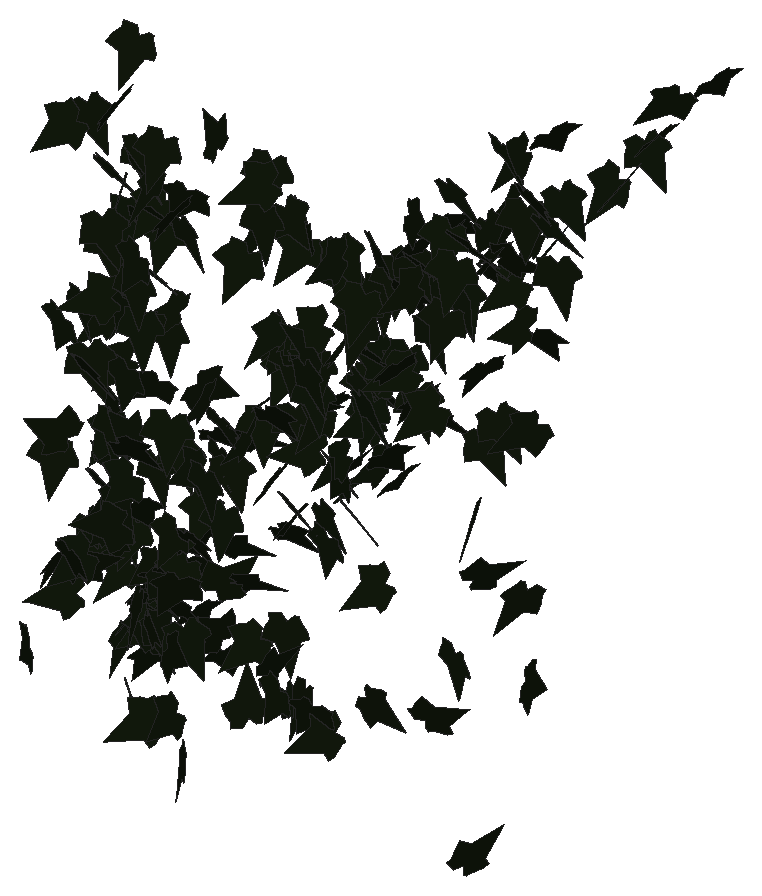
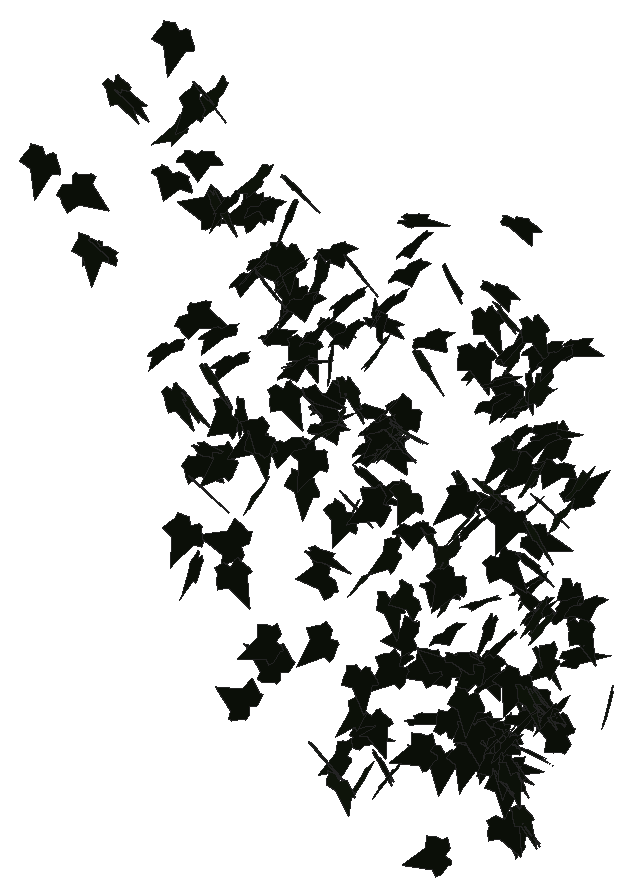
# SketchUp Ruby script. Lengths in inches.
U = 1.inch
M = Sketchup.active_model
def pt(a) = Geom::Point3d.new(a.map { |v| v * U })
def face(e, loops, mat)
  f = e.add_face(loops[0].map { |a| pt(a) })
  loops[1..].each { |l| e.add_face(l.map { |a| pt(a) }).erase! }
  f.material = f.back_material = mat if mat
  f
end
# faces: each face lists its corners as indices into pts; further lists are holes
def faces(e, pts, list, mat = nil) = list.each { |f| face(e, (f[0].is_a?(Array) ? f : [f]).map { |l| l.map { |i| pts[i] } }, mat) }
# xy, xz, yz: faces in a plane at the given z, y or x. An outline is a flat list of corners, or four numbers for a rectangle; further outlines are holes
def ring(l) = l.size == 4 ? [[l[0], l[1]], [l[2], l[1]], [l[2], l[3]], [l[0], l[3]]] : l.each_slice(2).to_a
def flat(e, list, mat, &to3) = list.each { |f| face(e, (f[0].is_a?(Array) ? f : [f]).map { |l| ring(l).map { |u, v| to3.(u, v) } }, mat) }
def xy(e, z, list, mat = nil) = flat(e, list, mat) { |x, y| [x, y, z] }
def xz(e, y, list, mat = nil) = flat(e, list, mat) { |x, z| [x, y, z] }
def yz(e, x, list, mat = nil) = flat(e, list, mat) { |y, z| [x, y, z] }
def lines(e, pts, list) = list.each { |a, b| e.add_line(pt(pts[a]), pt(pts[b])) }
# prism: a flat outline (further loops are holes) pulled along v
def prism(e, loops, v, mat = nil)
  f = face(e, loops, mat); d = Geom::Vector3d.new(v.map { |x| x * U })
  f.pushpull(f.normal.samedirection?(d) ? d.length : -d.length)
end
def box(e, o, s, mat = nil) = prism(e, [[o, [o[0] + s[0], o[1], o[2]], [o[0] + s[0], o[1] + s[1], o[2]], [o[0], o[1] + s[1], o[2]]]], [0, 0, s[2]], mat)
def at(x, y, z, deg = 0) = Geom::Transformation.translation(pt([x, y, z])) * Geom::Transformation.rotation(ORIGIN, Z_AXIS, deg.degrees)
def axes(o, x, y, z) = Geom::Transformation.new([*x, 0, *y, 0, *z, 0, *pt(o).to_a, 1])
def part(name) = M.definitions.add(name)
# library, detail: a bought-in or finely detailed component or shape, given as its bounding box
def library(name, o, s) = part(name).tap { |d| box(d.entities, o, s) }
def detail(e, o, s) = box(e.add_group.entities, o, s)
def put(e, d, t, mat = nil) = e.add_instance(d, t).tap { |i| i.material = mat if mat }
def group(e, t, mat = nil) = e.add_group.tap { |g| g.transformation = t; g.material = mat if mat }.entities
root = M.entities
M.materials.add("efeu1").color = [18, 25, 13]
c1 = part("ivyleaf_9")
p = [[1.54,2.16,1.25],[1.36,2.04,1.19],[-0.21,0.99,0.68],[-0.71,1.11,0.82],[-0.85,0.86,0.67],[-0.8,0.17,0.21],
  [-0.9,-0.01,0.1],[-0.67,-0.16,-0.02],[-0.08,-0.08,-0.05],[-0.03,-0.6,-0.4],[0.65,-0.88,-0.66],[0.83,-0.6,-0.49],
  [1.29,-0.42,-0.43],[1.8125,-0.07,-0.26],[1.21,0.44,0.15]]
faces(c1.entities,p,[[0,1,2,3,4,5,6,7,8,9,10,11,12,13,14]],"efeu1")
put(root,c1,axes([656.24,122.11,335.02],[-0.71022,1.11665,-0.15151],[0.0503,-0.14751,-1.32287],[-1.12576,-0.71106,0.03648]))
put(root,c1,axes([656.28,114.59,383.84],[-1.00018,-0.83735,0.69377],[-0.54915,-0.42464,-1.3042],[0.93857,-1.14077,-0.02376]))
put(root,c1,axes([655.3125,117.78,345.35],[0.65695,-1.07778,-0.75279],[-0.21372,0.74279,-1.24998],[1.29716,0.66822,0.1753]))
put(root,c1,axes([655.89,121.85,333.43],[-1.01827,-0.15161,-0.85733],[0.8683,-0.27334,-0.98296],[-0.06368,-1.30275,0.30601]))
put(root,c1,axes([655.37,116.96,366.04],[0.34286,-1.26926,0.60559],[0.26805,-0.55292,-1.31063],[1.38055,0.42258,0.10408]))
put(root,c1,axes([655.04,116.78,341.77],[0.99807,0.54618,-0.89303],[0.59041,0.7252,1.10339],[0.86443,-1.12594,0.27748]))
put(root,c1,axes([655.93,112.92,354.41],[-0.44767,-1.43357,-0.10005],[0.02948,0.09561,-1.50184],[1.43676,-0.44864,-0.00035]))
put(root,c1,axes([656.02,116.79,384.34],[0.25998,-1.28733,-0.70574],[-0.04875,0.70875,-1.31079],[1.46728,0.25164,0.08149]))
put(root,c1,axes([656.93,118.92,345],[-1.19552,-0.67601,0.07235],[-0.03238,-0.08956,-1.37202],[0.6791,-1.19436,0.06194]))
put(root,c1,axes([655.97,119.44,356.38],[1.06878,-0.9039,-0.24977],[-0.2235,0.12227,-1.39886],[0.91075,1.09074,-0.05018]))
put(root,c1,axes([657.5,117.57,345.86],[-1.23788,0.59991,-0.12376],[0.09621,-0.08516,-1.37516],[-0.60494,-1.24114,0.03453]))
put(root,c1,axes([656.03,134.68,335.79],[1.07083,0.22816,0.82919],[0.79435,0.24505,-1.09327],[-0.32956,1.33199,0.0591]))
put(root,c1,axes([658.09,117.64,345.03],[-0.32565,0.33631,-1.32818],[-1.11303,-0.86102,0.05488],[-0.79895,1.06242,0.46491]))
put(root,c1,axes([656.29,117.14,350.09],[1.35102,-0.32608,-0.00191],[-0.00104,0.00383,-1.38981],[0.32608,1.35102,0.00348]))
put(root,c1,axes([657.69,118.04,345.98],[-1.08082,0.8425,-0.16461],[0.12152,-0.11184,-1.37033],[-0.84978,-1.08755,0.0134]))
put(root,c1,axes([657.45,120.125,340.79],[-1.34084,-0.32062,-0.13981],[0.2222,-0.35305,-1.32142],[0.27012,-1.30105,0.39303]))
put(root,c1,axes([657.78,119.51,346.84],[-0.73022,1.16159,0.10689],[-0.05352,0.09262,-1.37204],[-1.16527,-0.73217,-0.00397]))
put(root,c1,axes([657.84,118.625,364.92],[-1.13991,0.87237,0.01427],[0.01406,0.04184,-1.43481],[-0.87238,-1.13923,-0.04177]))
put(root,c1,axes([656.69,120.92,344.59],[0.29639,-1.33638,-0.06778],[0.00877,0.07137,-1.36864],[1.33807,0.29555,0.02398]))
put(root,c1,axes([657.06,112.25,366.8],[-0.12136,-1.0892,1.01192],[0.30145,-1.01222,-1.05337],[1.45584,0.1188,0.30247]))
put(root,c1,axes([658.18,121.28,338.84],[-0.39023,1.27902,-0.09719],[0.01077,-0.09831,-1.33709],[-1.28266,-0.38995,0.01834]))
put(root,c1,axes([657.43,107.34,338.91],[0.04723,-0.43721,1.3925],[0.06038,-1.39145,-0.43893],[1.45827,0.07177,-0.02692]))
put(root,c1,axes([657.91,120.46,344.6],[-0.77173,-1.13212,-0.03722],[0.04554,0.01399,-1.36981],[1.13182,-0.7725,0.02973]))
put(root,c1,axes([658.65,115.96,349.41],[-0.98779,0.96189,-0.18111],[0.13218,-0.12386,-1.37875],[-0.96982,-0.99659,-0.00345]))
put(root,c1,axes([657.99,117.75,354.74],[-0.54169,-1.13622,0.61477],[-0.15612,-0.60416,-1.25418],[1.28241,-0.55349,0.107]))
put(root,c1,axes([658.32,121.66,337.93],[0.48242,1.21405,-0.3295],[-0.1248,-0.30497,-1.30638],[-1.25177,0.49829,0.00326]))
put(root,c1,axes([658.9,118.3,361.04],[-1.42192,0.17774,0.05329],[-0.0556,-0.01523,-1.43281],[-0.17703,-1.42283,0.022]))
put(root,c1,axes([657.73,117.9375,355.5],[0.08364,-1.39785,0.08215],[-0.01645,-0.08327,-1.40018],[1.40016,0.08253,-0.02136]))
put(root,c1,axes([659.01,115.96,366.48],[-1.42993,0.25709,-0.07317],[0.04156,-0.17951,-1.44299],[-0.26404,-1.42051,0.16911]))
put(root,c1,axes([658.87,121.53,332.9],[0.01974,1.02003,-0.88375],[-0.14459,-0.87716,-1.01566],[-1.34186,0.10952,0.09644]))
put(root,c1,axes([657.73,116.39,379.9],[1.33733,-0.63028,-0.0417],[0.06152,0.22713,-1.46016],[0.62865,1.31856,0.23159]))
put(root,c1,axes([657.78,116.74,352.91],[0.62527,-1.2148,0.28921],[0.21503,-0.21386,-1.36322],[1.2301,0.65488,0.0913]))
put(root,c1,axes([658.76,122.36,337.74],[-1.09637,-0.26636,-0.72385],[0.74209,-0.02137,-1.11614],[0.21024,-1.31359,0.16494]))
put(root,c1,axes([659.14,121.8,339.61],[0.71264,0.8805,-0.72368],[-0.45012,-0.56669,-1.13274],[-1.04709,0.84287,-0.00559]))
put(root,c1,axes([659.58,116.03,386.12],[-0.62586,1.32112,-0.36173],[0.13171,-0.33782,-1.46166],[-1.3634,-0.63908,0.02485]))
put(root,c1,axes([658.25,134.16,346.49],[1.00881,0.33998,0.83846],[0.7427,0.40602,-1.05823],[-0.51672,1.24734,0.11593]))
put(root,c1,axes([658.53,116.38,373.48],[-0.10525,-1.44792,-0.35467],[0.21802,0.33678,-1.43958],[1.4747,-0.15313,0.18752]))
put(root,c1,axes([659.14,118.82,347.63],[0.94591,0.99244,-0.16489],[-0.11204,-0.121,-1.37101],[-0.99978,0.95252,-0.00236]))
put(root,c1,axes([659.06,121.66,341.04],[0.37215,-0.59504,-1.15024],[0.59763,-0.98283,0.70179],[-1.1489,-0.70399,-0.00753]))
put(root,c1,axes([660.35,119.15,337.49],[-0.9,0.89881,0.43769],[-0.35351,0.26475,-1.27058],[-0.93513,-0.96513,0.05907]))
put(root,c1,axes([658.89,119.1,328.8],[-0.15229,-0.16631,1.41236],[0.40306,-1.36724,-0.11753],[1.3638,0.38551,0.19245]))
put(root,c1,axes([659.97,120.03,341.08],[0.58504,1.21298,-0.06639],[-0.14393,-0.00395,-1.34062],[-1.20624,0.58878,0.12777]))
put(root,c1,axes([660.34,107.78,348.32],[-0.56945,1.20528,-0.58163],[0.25936,-0.52072,-1.33299],[-1.31291,-0.62563,-0.01105]))
put(root,c1,axes([661.02,116.12,355.15],[-0.27991,0.4357,1.38305],[-0.9607,0.99937,-0.50926],[-1.08615,-0.99622,0.09402]))
put(root,c1,axes([661.125,108.58,344.625],[-0.89995,-0.31747,1.08852],[-0.93011,-0.58814,-0.94051],[0.64851,-1.28409,0.16165]))
put(root,c1,axes([661.1,119.17,337.36],[-1.31357,-0.20553,0.30416],[-0.29593,-0.0758,-1.32925],[0.21721,-1.34619,0.02841]))
put(root,c1,axes([660.32,118.36,365.46],[1.02839,0.989,-0.20213],[-0.16985,-0.1149,-1.42636],[-0.99505,1.04175,0.03457]))
put(root,c1,axes([659.83,116.28,368.03],[0.05204,-1.12236,0.94769],[0.22028,-0.9316,-1.1154],[1.45233,0.18151,0.13522]))
put(root,c1,axes([660.18,116.09,378.82],[-0.63713,0.12987,-1.35187],[1.18093,-0.68446,-0.62232],[-0.6707,-1.32854,0.18847]))
put(root,c1,axes([660.57,121.2,340.62],[1.18084,0.30799,-0.57443],[-0.55151,-0.16135,-1.22025],[-0.34736,1.30319,-0.01532]))
put(root,c1,axes([661.71,118.53,360.02],[0.04728,0.67777,-1.2711],[-0.8779,-0.99476,-0.56307],[-1.14209,0.79271,0.38021]))
put(root,c1,axes([660.45,120.5,340.84],[0.5226,-1.11443,-0.62384],[-0.30285,0.54669,-1.23031],[1.24073,0.60284,-0.03755]))
put(root,c1,axes([660.5,119.97,351.72],[0.23802,-1.37389,-0.11875],[-0.00334,0.11993,-1.39425],[1.37901,0.23743,0.01712]))
put(root,c1,axes([661.4375,115.52,376.19],[-0.75501,-0.51266,1.16043],[-0.61135,-1.03622,-0.85555],[1.11161,-0.91809,0.31765]))
put(root,c1,axes([662.24,111.69,370.9],[-0.98534,-0.3661,1.03841],[-0.92225,-0.48682,-1.04675],[0.60148,-1.34618,0.09614]))
put(root,c1,axes([662.32,121.78,342.32],[0.59601,0.91809,-0.79993],[-0.47504,-0.64474,-1.09392],[-1.12121,0.7612,0.03825]))
put(root,c1,axes([662.61,105.65,360.88],[0.06608,0.00927,1.487],[-1.30235,-0.71808,0.06235],[0.71775,-1.3038,-0.02377]))
put(root,c1,axes([662.97,117.75,336.88],[-0.31482,0.56395,1.19527],[-0.62339,1.02008,-0.64549],[-1.16537,-0.69802,0.02239]))
put(root,c1,axes([661.74,116.84,371.39],[1.40626,0.06522,-0.35296],[-0.35893,0.25859,-1.38228],[0.00077,1.42664,0.26669]))
put(root,c1,axes([661.72,109.78,366.71],[-0.44533,-0.97085,-0.99995],[0.60222,0.81266,-1.05721],[1.2569,-0.73336,0.15225]))
put(root,c1,axes([661.92,116.23,382.97],[0.28141,-1.45855,-0.25764],[-0.02711,0.25713,-1.48529],[1.48088,0.28187,0.02176]))
put(root,c1,axes([662.8,107.89,349.1],[-0.68649,-1.02408,0.86523],[-0.51555,-0.69567,-1.23243],[1.23757,-0.85787,-0.03345]))
put(root,c1,axes([662.6,121.08,342.36],[-0.76681,-1.11957,0.1339],[0.06958,-0.20861,-1.34574],[1.1254,-0.74994,0.17444]))
put(root,c1,axes([662.09,114.28,362.9375],[-0.07596,-1.30748,0.69233],[0.22601,-0.69536,-1.2884],[1.4621,0.03956,0.23513]))
put(root,c1,axes([661.83,115.63,381.96],[1.0101,-1.08977,0.30654],[0.19895,-0.23354,-1.48585],[1.11444,1.02943,-0.01258]))
put(root,c1,axes([663.1,105.48,350.45],[1.02888,0.12155,-1.068],[-1.05239,-0.18705,-1.03512],[-0.21882,1.47113,-0.04337]))
put(root,c1,axes([662.72,119.62,346.17],[-0.34674,-1.19087,0.54912],[-0.05103,-0.55531,-1.23651],[1.31038,-0.33674,0.09715]))
put(root,c1,axes([664.06,118.16,367.33],[-1.07535,0.89327,0.40312],[-0.51318,-0.00338,-1.36142],[-0.83492,-1.14842,0.31757]))
put(root,c1,axes([662.98,115.95,339.75],[0.92926,-0.61503,-0.92823],[-0.78505,0.49552,-1.11425],[0.78966,1.21639,-0.01542]))
put(root,c1,axes([662.81,115.22,377.53],[1.3823,0.44114,-0.2309],[-0.20323,-0.12215,-1.44998],[-0.45456,1.39612,-0.0539]))
put(root,c1,axes([663.18,113.34,354],[-0.70217,-0.99335,0.81584],[-0.082,-0.89311,-1.15801],[1.28281,-0.60082,0.37254]))
put(root,c1,axes([663.6,121.18,344.95],[0.16122,1.35312,0.00386],[-0.00695,0.00472,-1.36267],[-1.3531,0.16119,0.00746]))
put(root,c1,axes([663.09,114.44,342.43],[-0.86043,0.19228,-1.18489],[1.13792,-0.3335,-0.88044],[-0.38219,-1.42585,0.04614]))
put(root,c1,axes([662.71,116.89,338.54],[0.70332,-1.23211,-0.24038],[-0.06295,0.24058,-1.41729],[1.25377,0.70326,0.06369]))
put(root,c1,axes([663.62,121,338.39],[0.41196,1.29916,0.1099],[0.01709,0.10986,-1.3628],[-1.30368,0.41197,0.01686]))
put(root,c1,axes([662.73,116.16,339.12],[0.12761,-0.14919,-1.46844],[0.78281,1.25639,-0.05962],[1.25131,-0.77077,0.18705]))
put(root,c1,axes([663.22,111.26,353.46],[0.56013,-1.27597,-0.4935],[-0.17754,0.46096,-1.39334],[1.35651,0.58721,0.02142]))
put(root,c1,axes([663.31,109.63,379.4],[-0.16267,-1.21915,-0.82843],[0.18214,0.81045,-1.22845],[1.46269,-0.2365,0.06083]))
put(root,c1,axes([663.91,116.62,378.26],[-0.97547,-1.0603,0.3972],[0.00977,-0.53214,-1.39653],[1.13222,-0.90892,0.35426]))
put(root,c1,axes([664.05,113.17,394.9],[-1.24292,-0.72594,-0.4531],[0.41408,0.18901,-1.43873],[0.74888,-1.30936,0.04353]))
put(root,c1,axes([663.55,117.79,366.0625],[0.08239,-1.44543,0.00768],[-0.00012,-0.0077,-1.44778],[1.44545,0.08239,-0.00056]))
put(root,c1,axes([663.45,106.53,367.71],[1.46369,-0.23984,-0.10882],[-0.10653,0.02287,-1.4832],[0.24087,1.46755,0.00533]))
put(root,c1,axes([664.2,116.85,376.14],[-0.5692,-1.36042,-0.02757],[0.01401,0.02402,-1.47469],[1.36063,-0.56936,0.00365]))
put(root,c1,axes([663.52,118.34,340.21],[1.29631,-0.13381,0.40419],[0.3974,-0.08464,-1.30254],[0.15281,1.35522,-0.04144]))
put(root,c1,axes([663.97,118.82,354.62],[-0.09444,-1.36865,-0.28529],[0.4693,0.23831,-1.29865],[1.31695,-0.18307,0.44232]))
put(root,c1,axes([665.46,139.01,342.58],[-0.31265,1.26804,0.49947],[-0.38546,0.40925,-1.28027],[-1.30722,-0.42396,0.25805]))
put(root,c1,axes([665.7,113.03,332.65],[-1.00224,-0.64191,0.88595],[-0.74555,-0.47861,-1.19018],[0.8007,-1.24913,0.00074]))
put(root,c1,axes([665.18,120.88,348.89],[-1.10702,-0.75937,-0.27754],[0.24848,0.12824,-1.34201],[0.76937,-1.13406,0.03408]))
put(root,c1,axes([664.79,118.6,346.85],[1.32731,0.14047,-0.29244],[-0.29444,0.00441,-1.33428],[-0.13622,1.35914,0.03455]))
put(root,c1,axes([664.72,112.09,373.45],[0.12411,-1.49888,0.06118],[0.00981,-0.06058,-1.504],[1.50009,0.1244,0.00477]))
put(root,c1,axes([665.3,112.2,369.84],[-0.1163,-1.4569,-0.19574],[-0.0193,0.19784,-1.46112],[1.46986,-0.11267,-0.03467]))
put(root,c1,axes([665.11,135.52,341.9],[0.94467,-0.96542,-0.37035],[-0.23925,0.28395,-1.35045],[1.00596,0.97413,0.02661]))
put(root,c1,axes([666.43,134.57,352.54],[0.00011,1.35101,-0.22901],[-0.00973,-0.229,-1.35098],[-1.37025,0.00173,0.00957]))
put(root,c1,axes([666.87,115.92,380.45],[0.6346,0.68927,-1.1747],[-0.86756,-0.79445,-0.93483],[-1.04992,1.07307,0.06244]))
put(root,c1,axes([666.68,112.26,383.33],[-1.27244,0.03999,-0.77222],[0.72909,-0.43331,-1.22381],[-0.25759,-1.42397,0.35072]))
put(root,c1,axes([667.06,114.63,345.14],[0.43516,0.87156,-1.14125],[-0.51255,-1.01969,-0.97416],[-1.34141,0.67236,0.002]))
put(root,c1,axes([666.82,112.94,386.36],[-1.23419,-0.65133,-0.55971],[0.52629,0.20073,-1.39408],[0.67862,-1.34023,0.06322]))
put(root,c1,axes([666.89,114.34,333.04],[-0.35376,-0.93984,0.94769],[-0.34332,-0.88335,-1.00419],[1.28979,-0.49291,-0.00737]))
put(root,c1,axes([666.78,119.64,356.67],[1.03272,0.91922,0.01181],[-0.09536,0.12479,-1.37366],[-0.91434,1.02522,0.15661]))
put(root,c1,axes([668.12,105.72,354.7],[-0.50351,-0.19864,-1.4024],[-0.91591,-1.08965,0.48319],[-1.08041,1.01632,0.24395]))
put(root,c1,axes([666.65,120.41,354.5],[0.53181,-1.13037,0.60093],[0.24283,-0.54984,-1.24915],[1.25693,0.58449,-0.01293]))
put(root,c1,axes([667.61,120.02,336.54],[0.64365,1.16256,-0.35129],[-0.18118,-0.30121,-1.32879],[-1.20088,0.66856,0.01219]))
put(root,c1,axes([668.3,139.38,345.58],[-1.23118,0.66709,0.14111],[-0.15604,0.00788,-1.39868],[-0.66375,-1.23922,0.06707]))
put(root,c1,axes([666.99,133.99,347.92],[1.29193,-0.4425,-0.15002],[-0.14948,0.02648,-1.36541],[0.44269,1.30034,-0.02324]))
put(root,c1,axes([667.5,108.85,377.7],[-0.16729,-1.1428,0.94464],[-0.04326,-0.94647,-1.15267],[1.48204,-0.15663,0.07298]))
put(root,c1,axes([667.32,114.73,378.19],[0.8746,-1.19951,0.10159],[0.05744,-0.08385,-1.48451],[1.20244,0.87648,-0.00298]))
put(root,c1,axes([668.31,118.54,338.65],[0.29865,0.37267,1.35675],[-0.91662,-1.00073,0.47665],[1.06745,-0.96359,0.0297]))
put(root,c1,axes([668.12,119.29,349.81],[-0.21022,-1.37384,0.06285],[-0.01101,-0.0619,-1.38983],[1.37524,-0.2105,-0.00152]))
put(root,c1,axes([667.62,135.38,343.19],[1.27815,-0.57149,0.1111],[0.09992,-0.04871,-1.40009],[0.57355,1.28205,-0.00367]))
put(root,c1,axes([667.74,119.16,358.34],[0.46389,-1.1148,0.75016],[0.58947,-0.54433,-1.17343],[1.20749,0.694,0.28465]))
put(root,c1,axes([668.48,111.84,361.6],[-0.88555,-1.00647,-0.67325],[0.50059,0.45518,-1.33891],[1.10257,-1.01502,0.06716]))
put(root,c1,axes([669.32,111.22,381.55],[-0.49822,1.35036,-0.44056],[0.08692,-0.43701,-1.43779],[-1.41775,-0.50133,0.06667]))
put(root,c1,axes([668.625,115.34,363.58],[-0.00142,0.02126,-1.50798],[-0.32785,1.47191,0.02106],[1.47206,0.32783,0.00324]))
put(root,c1,axes([668.63,105.33,362.45],[1.39941,0.44335,0.25844],[0.25063,0.06456,-1.46789],[-0.44781,1.42161,-0.01393]))
put(root,c1,axes([668.84,119.08,354.7],[-0.52267,-0.90994,-0.91845],[0.66601,0.65961,-1.03251],[1.10814,-0.82562,0.18735]))
put(root,c1,axes([668.9,117.48,343.95],[-0.29257,-0.08966,1.44092],[1.43709,0.12258,0.29942],[-0.13813,1.46521,0.06312]))
put(root,c1,axes([670.64,115.05,386.39],[-0.18221,0.4928,1.41934],[-0.68271,1.24646,-0.52041],[-1.33839,-0.7029,0.07223]))
put(root,c1,axes([669.25,112.65,342.33],[0.04753,-1.27417,-0.81821],[0.10665,0.81939,-1.26983],[1.5105,-0.01776,0.1154]))
put(root,c1,axes([670.85,113.59,363.75],[-1.08423,0.91326,-0.10998],[0.11169,-0.03803,-1.41695],[-0.91305,-1.08913,-0.04274]))
put(root,c1,axes([670.59,113.07,357.39],[-0.48668,-0.5933,1.17746],[-0.42486,-1.11759,-0.73875],[1.24816,-0.61176,0.20764]))
put(root,c1,axes([669.96,135.27,355.4375],[1.4119,0.21932,0.16636],[0.1691,-0.00502,-1.4285],[-0.21721,1.42165,-0.03071]))
put(root,c1,axes([671.34,119.49,339.15],[-1.11615,-0.75953,0.46039],[-0.22075,-0.47895,-1.32533],[0.8603,-1.10831,0.25722]))
put(root,c1,axes([670.39,111.06,331.95],[-0.10898,-0.10367,-1.49281],[1.34171,-0.66953,-0.05145],[-0.6626,-1.33869,0.14134]))
put(root,c1,axes([670.45,123.74,347.14],[1.28893,0.42182,0.2362],[0.22494,0.0721,-1.3562],[-0.42793,1.30841,-0.00142]))
put(root,c1,axes([670.375,118.24,344.74],[1.14751,0.12093,0.76479],[0.71684,0.35092,-1.13106],[-0.29267,1.33362,0.22827]))
put(root,c1,axes([671.7,120.03,353.01],[-0.56571,0.91721,-0.8899],[-0.4649,0.75881,1.07763],[1.1904,0.73222,-0.00205]))
put(root,c1,axes([672.23,117.17,359.2],[-1.16196,0.81927,-0.14576],[0.1326,-0.06485,-1.42155],[-0.8215,-1.16927,-0.02328]))
put(root,c1,axes([672.13,117.29,333.37],[-1.46373,0.17302,0.11325],[0.11165,-0.02018,1.4739],[0.17405,1.46797,0.00692]))
put(root,c1,axes([672.24,106.84,344.08],[0.40729,-0.21936,-1.35694],[-1.00681,0.91591,-0.45026],[0.93581,1.08087,0.10615]))
put(root,c1,axes([671.43,112.63,357.36],[0.33715,-1.36506,0.4324],[0.17789,-0.40085,-1.40417],[1.42081,0.37411,0.0732]))
put(root,c1,axes([673.18,116.74,377.875],[-1.12197,0.97288,0.0186],[-0.01502,0.01107,-1.48503],[-0.97294,-1.12207,0.00147]))
put(root,c1,axes([672.29,119.24,360.19],[-0.64256,-1.13933,-0.53327],[0.28644,0.45057,-1.30777],[1.22491,-0.70303,0.02608]))
put(root,c1,axes([672.7,121.66,333.67],[0.78028,-1.03601,-0.56814],[-0.23815,0.52897,-1.29167],[1.15732,0.80735,0.11725]))
put(root,c1,axes([673.57,117.79,362.8],[0.36663,1.20329,0.62989],[-0.11405,0.67741,-1.22767],[-1.35339,0.26888,0.2741]))
put(root,c1,axes([674.65,119.65,351.29],[-0.38179,1.35449,0.05648],[0.00163,0.05914,-1.40716],[-1.35566,-0.38138,-0.0176]))
put(root,c1,axes([674.28,121.76,334.43],[-1.12671,0.02339,-0.86278],[0.86043,-0.08103,-1.12584],[-0.06781,-1.41679,0.05015]))
put(root,c1,axes([674.66,117.98,369.78],[-1.36501,-0.32845,-0.38418],[0.47905,-0.48787,-1.28499],[0.16119,-1.33147,0.56561]))
put(root,c1,axes([674.7,113.78,378.28],[-0.84871,-1.22771,0.1124],[-0.0527,-0.1002,-1.49245],[1.23172,-0.85023,0.01359]))
put(root,c1,axes([675.41,117.48,367.55],[-1.34534,0.39426,-0.44857],[-0.43158,0.12231,1.40191],[0.41278,1.41286,0.00381]))
put(root,c1,axes([675.83,118.24,366.86],[-1.17799,-0.77493,-0.29532],[0.2781,0.11417,-1.4089],[0.78128,-1.20906,0.05624]))
put(root,c1,axes([675.53,118.55,367.76],[0.02575,-1.44015,0.00221],[-0.00013,-0.00222,-1.44038],[1.44015,0.02575,-0.00017]))
put(root,c1,axes([675.82,115.63,386.38],[-0.37654,-1.45468,-0.11155],[0.01829,0.11049,-1.50259],[1.45884,-0.37685,-0.00995]))
put(root,c1,axes([675.7,117.8,342.86],[0.01371,-1.50693,-0.15959],[-0.0059,0.15954,-1.50698],[1.51534,0.01425,-0.00442]))
put(root,c1,axes([675.43,118.56,368.02],[0.83246,-1.1673,-0.14836],[0.04941,0.21625,-1.42421],[1.17565,0.81746,0.16491]))
put(root,c1,axes([675.77,119.71,361.79],[0.78313,0.78513,0.86915],[0.57113,0.65683,-1.10794],[-1.02257,0.96814,0.04682]))
put(root,c1,axes([675.47,136.87,353.88],[1.3688,-0.08112,0.44483],[0.44793,0.04947,-1.3693],[0.06179,1.43842,0.07217]))
put(root,c1,axes([675.81,118.375,368.74],[0.01131,-0.87813,-1.1424],[0.5321,1.06423,-0.81278],[1.33906,-0.41548,0.33262]))
put(root,c1,axes([676.45,117.96,362.65],[-0.17814,-1.23294,-0.6519],[0.11786,0.64154,-1.24555],[1.38969,-0.21246,0.02207]))
put(root,c1,axes([676.21,116.91,354.97],[1.33424,-0.45883,0.00894],[0.00833,-0.00327,-1.41093],[0.45884,1.33427,-0.00038]))
put(root,c1,axes([677.02,118.5,369.85],[0.07812,-1.30015,-0.61932],[-0.03023,0.61862,-1.30248],[1.43981,0.08353,0.00626]))
put(root,c1,axes([676.73,117.79,367.65],[1.00391,-0.97791,0.29204],[0.17373,-0.23992,-1.4006],[1.00569,1.01762,-0.04957]))
put(root,c1,axes([678.3,117.87,336.01],[0.56024,0.66093,-1.12253],[-0.85635,-0.73394,-0.85952],[-0.98161,1.01749,0.10917]))
put(root,c1,axes([678.53,118.63,370.95],[-1.34554,-0.20134,0.42441],[-0.40252,-0.16956,-1.3566],[0.24214,-1.40066,0.10322]))
put(root,c1,axes([677.34,115.67,382.625],[0.57418,-1.11601,-0.85183],[-0.15696,0.86352,-1.23712],[1.39515,0.55645,0.2114]))
put(root,c1,axes([678.36,118.15,368.72],[0.02504,-1.45181,-0.02128],[-0.0151,-0.02154,1.45194],[-1.45189,-0.02482,-0.01546]))
put(root,c1,axes([678.84,116.51,379.3],[0.13508,-0.33713,1.45485],[-0.5289,1.35531,0.36318],[-1.39661,-0.54587,0.00318]))
put(root,c1,axes([679.35,117.02,360.39],[-1.11454,0.05815,0.86777],[-0.86921,-0.12262,-1.10817],[0.02969,-1.40719,0.13243]))
put(root,c1,axes([677.92,119,367.71],[-0.00489,-1.42792,-0.03492],[-0.05174,0.03507,-1.42698],[1.42741,-0.00362,-0.05184]))
put(root,c1,axes([678.89,116.36,379.91],[-1.32769,-0.69621,-0.03301],[0.1084,-0.13611,-1.48939],[0.68851,-1.3211,0.17085]))
put(root,c1,axes([678.53,111.45,342.07],[0.21363,0.32781,1.36881],[0.82754,1.09066,-0.39035],[-1.13854,0.85425,-0.02689]))
put(root,c1,axes([679.61,118.8125,333.75],[-0.91794,-0.61078,0.9107],[-0.78677,-0.46044,-1.10182],[0.76382,-1.2083,-0.04048]))
put(root,c1,axes([679.38,118.11,363.52],[-1.39606,-0.08857,-0.26621],[0.26777,-0.01731,-1.39846],[0.08374,-1.42111,0.03362]))
put(root,c1,axes([679.85,110.3,388.22],[-1.25185,-0.35015,0.73544],[-0.60718,-0.49772,-1.27051],[0.54296,-1.36391,0.27483]))
put(root,c1,axes([678.6,117.67,365.8],[0.0055,-1.40369,-0.17962],[0.13257,0.17934,-1.39746],[1.40891,-0.01139,0.1322]))
put(root,c1,axes([680.03,133.25,373.49],[-0.27223,1.43082,-0.02284],[0.00414,-0.02246,-1.45649],[-1.43099,-0.27227,0.00013]))
put(root,c1,axes([678.98,118.95,351.3],[0.04406,-1.23369,0.69336],[0.21956,-0.67934,-1.2227],[1.39805,0.14557,0.17017]))
put(root,c1,axes([679.49,110.54,366.97],[1.34951,0.48708,-0.11313],[-0.10485,-0.04275,-1.43472],[-0.48893,1.35357,-0.0046]))
put(root,c1,axes([679.5,109.99,385.54],[0.07756,-1.48528,-0.01857],[-0.00149,0.01852,-1.4873],[1.48539,0.07758,-0.00052]))
put(root,c1,axes([679.5,133.45,374.28],[1.10304,0.70408,0.61716],[0.49211,0.37536,-1.30776],[-0.79653,1.20693,0.04669]))
put(root,c1,axes([680.87,136.76,360.2],[-0.27339,1.23285,-0.73202],[-0.01833,-0.74815,-1.25318],[-1.43368,-0.22553,0.15561]))
put(root,c1,axes([680.16,111.16,341.09],[-0.13737,-1.06306,0.94263],[0.01758,-0.94823,-1.06681],[1.42068,-0.09106,0.10434]))
put(root,c1,axes([681.19,118.32,359.98],[-1.37112,0.32287,-0.19373],[0.17402,-0.10538,-1.40725],[-0.3339,-1.38072,0.0621]))
put(root,c1,axes([680.88,118.96,358.54],[0.28734,1.26951,0.59267],[-0.02009,0.60868,-1.29406],[-1.40089,0.25166,0.14013]))
put(root,c1,axes([680.3,118.91,358.09],[0.62542,-0.46193,-1.19881],[0.96477,-0.71158,0.77752],[-0.84837,-1.14976,0.00043]))
put(root,c1,axes([682.49,116.6,371.56],[-0.80872,1.1905,-0.05372],[0.03193,-0.04325,-1.43921],[-1.19129,-0.80935,-0.0021]))
put(root,c1,axes([682.1,117.38,377.91],[-0.11883,-1.46967,-0.03001],[-0.0447,0.03371,-1.4737],[1.46929,-0.11784,-0.04726]))
put(root,c1,axes([682.66,115.95,381.07],[0.35653,-1.32377,-0.64662],[0.01216,0.6679,-1.36064],[1.4732,0.31485,0.16772]))
put(root,c1,axes([682.67,117.93,368.04],[1.2083,-0.61085,-0.49034],[-0.16351,0.68487,-1.2561],[0.76606,1.10967,0.50532]))
put(root,c1,axes([683.35,119.23,367.65],[-0.94104,-1.04549,-0.26852],[0.27427,0.11295,-1.40097],[1.044,-0.97206,0.12601]))
put(root,c1,axes([682.25,118.74,369.95],[0.8011,-0.44513,1.10199],[0.96834,-0.52605,-0.91644],[0.68908,1.25674,0.00672]))
put(root,c1,axes([683,134.51,370.8],[1.42881,-0.04326,0.00196],[0.00201,0.00172,-1.42946],[0.04325,1.42881,0.00178]))
put(root,c1,axes([684.87,118.73,369.65],[-0.45656,0.23798,1.34108],[-1.16643,0.66199,-0.51457],[-0.70326,-1.25248,-0.01715]))
put(root,c1,axes([683.17,118.26,374.61],[0.11683,-0.05899,-1.44158],[1.36658,-0.45931,0.12954],[-0.4627,-1.37144,0.01862]))
put(root,c1,axes([683.37,110.56,372.3125],[0.7999,-1.2895,-0.02319],[-0.01295,0.01926,-1.51744],[1.28964,0.8,-0.00086]))
put(root,c1,axes([685.49,112.43,382.41],[-1.38242,0.54406,0.10607],[-0.08006,0.08604,-1.48476],[-0.54849,-1.38381,-0.05061]))
put(root,c1,axes([685.29,131.5,373.63],[0.31967,0.8956,1.13524],[0.27166,1.10475,-0.94804],[-1.42024,0.4129,0.07418]))
put(root,c1,axes([685.12,138.13,363.97],[1.19524,0.80782,-0.26787],[-0.25755,-0.09685,-1.44125],[-0.81117,1.22105,0.0629]))
put(root,c1,axes([685.61,116.66,365.72],[-0.7881,-0.63932,1.06645],[-0.47355,-1.01314,-0.95731],[1.14969,-0.85555,0.33673]))
put(root,c1,axes([686.39,134.42,370.85],[-1.40365,-0.19848,0.24245],[-0.23362,-0.07865,-1.41692],[0.2088,-1.42226,0.04452]))
put(root,c1,axes([685.2,118.125,377.31],[0.08793,-1.44975,0.03493],[0.00041,-0.03497,-1.45241],[1.45017,0.08791,-0.00171]))
put(root,c1,axes([685.76,116.29,367.33],[-1.13396,-0.57806,-0.70492],[0.69948,0.1698,-1.26445],[0.58464,-1.32437,0.14557]))
put(root,c1,axes([686.93,134.58,366.72],[-1.20442,0.71168,0.47101],[-0.47989,0.10892,-1.39169],[-0.70572,-1.28865,0.1425]))
put(root,c1,axes([686.74,116.36,351.01],[-1.39071,-0.15246,0.37946],[-0.37394,-0.07034,-1.39876],[0.16552,-1.43983,0.02815]))
put(root,c1,axes([686.6875,133.31,378.9375],[-1.12722,0.90564,-0.04749],[0.03552,-0.03161,-1.44597],[-0.90619,-1.12778,0.0024]))
put(root,c1,axes([686.07,114.47,376.0625],[-1.17132,-0.62663,-0.58884],[0.55416,0.21076,-1.3266],[0.65751,-1.29395,0.06909]))
put(root,c1,axes([686.65,118.15,359.875],[0.00273,1.42249,0.21712],[-0.0764,0.21696,-1.42047],[-1.43694,-0.00883,0.07594]))
put(root,c1,axes([685.96,122,366.01],[-0.25461,-1.25388,-0.64372],[0.15138,0.62603,-1.27929],[1.40131,-0.29545,0.02124]))
put(root,c1,axes([686.42,116.84,362.61],[0.65157,1.27703,0.1716],[0.09045,0.14649,-1.43358],[-1.28533,0.65768,-0.01389]))
put(root,c1,axes([685.72,114.88,368.41],[1.07513,-1.05416,-0.02386],[-0.01731,0.01642,-1.50571],[1.05429,1.07527,-0.0004]))
put(root,c1,axes([685.93,116.4,381.84],[0.95015,-0.44085,-1.07984],[0.99778,-0.41406,1.04698],[-0.60402,-1.37746,0.03087]))
put(root,c1,axes([687.27,117.76,379.83],[-0.45875,-1.3511,-0.31739],[0.05164,0.31744,-1.42591],[1.38692,-0.45872,-0.05189]))
put(root,c1,axes([688.05,134.7,375.51],[-1.27034,0.37642,-0.5762],[0.47277,-0.4018,-1.30481],[-0.50019,-1.33579,0.23011]))
put(root,c1,axes([688.01,117.98,372.22],[-0.18058,-1.44406,-0.07033],[0.00868,0.06979,-1.45531],[1.44574,-0.18079,-0.00005]))
put(root,c1,axes([689.24,116.65,371.45],[-1.20784,-0.45087,0.75555],[-0.42856,-0.81923,-1.17397],[0.76842,-1.16559,0.53287]))
put(root,c1,axes([689.5,117.76,368.82],[-0.36652,1.25461,-0.65412],[-0.01958,-0.68014,-1.29355],[-1.41475,-0.31562,0.18736]))
put(root,c1,axes([689.56,114.6,372.98],[-0.29331,1.32512,-0.53209],[0.00164,-0.54288,-1.35291],[-1.42795,-0.27281,0.10774]))
put(root,c1,axes([689.95,134.52,375.85],[-0.79705,1.11002,-0.49201],[0.20058,-0.46009,-1.36294],[-1.19749,-0.8159,0.09919]))
put(root,c1,axes([689.33,115.89,379.54],[1.30745,0.39742,-0.49683],[-0.50448,-0.04427,-1.363],[-0.38766,1.39797,0.09808]))
put(root,c1,axes([689.14,116.77,382.21],[0.44849,-1.274,-0.58163],[-0.02021,0.60478,-1.34028],[1.40034,0.41676,0.16693]))
put(root,c1,axes([689.66,110.18,381.35],[-0.73968,-1.26803,-0.14603],[0.08802,0.1177,-1.46791],[1.27337,-0.74471,0.01664]))
put(root,c1,axes([690.24,116.46,383.76],[0.0486,1.44248,-0.24604],[-0.07591,-0.24336,-1.44176],[-1.46134,0.06061,0.06671]))
put(root,c1,axes([689.13,119.08,338.14],[0.17849,-0.29107,1.44721],[1.44102,-0.28194,-0.23443],[0.32029,1.43066,0.24824]))
put(root,c1,axes([691.95,117.73,380.16],[-0.82814,0.82897,0.87674],[-0.62637,0.61351,-1.17173],[-1.03128,-1.03832,0.00764]))
put(root,c1,axes([691.1,114.42,387.42],[0.64143,-0.32697,-1.31555],[-1.01946,0.8429,-0.70657],[0.89346,1.19651,0.13825]))
put(root,c1,axes([689.98,116.42,381.8],[1.17874,-0.62645,0.68849],[0.71736,-0.09657,-1.31604],[0.59317,1.36166,0.22342]))
put(root,c1,axes([690.55,117.36,376.01],[0.63106,-1.31121,-0.15388],[-0.0333,0.15469,-1.4547],[1.31979,0.63086,0.03687]))
put(root,c1,axes([690.24,110.13,344.4],[0.20439,-0.07819,-1.43977],[1.2398,0.75197,0.13516],[0.73618,-1.24469,0.1721]))
put(root,c1,axes([690.83,134.27,380.69],[0.23896,-1.20813,-0.77838],[0.09026,0.80013,-1.21417],[1.43434,0.15092,0.20609]))
put(root,c1,axes([692.67,120.86,351.625],[0.49607,-0.06709,1.39867],[1.30091,0.57108,-0.434],[-0.51808,1.36975,0.24945]))
put(root,c1,axes([694.5625,113.36,371.37],[-1.19969,-0.73423,0.4595],[-0.37553,-0.26645,-1.40622],[0.78051,-1.25674,0.02969]))
put(root,c1,axes([694,117.6,380.31],[0.03698,-1.38947,-0.4731],[0.01983,0.47368,-1.38962],[1.46767,0.02861,0.03069]))
put(root,c1,axes([693.85,116.74,380.75],[0.5759,-1.33843,-0.24182],[-0.05417,0.23982,-1.45639],[1.35902,0.57673,0.04443]))
put(root,c1,axes([694.38,115.4,386.82],[-0.61937,-1.33704,0.0176],[-0.01142,-0.0141,-1.47353],[1.33711,-0.61946,-0.00443]))
put(root,c1,axes([693.75,116.04,390.36],[1.00825,-1.0814,0.05819],[0.25417,0.15901,-1.44897],[1.05272,0.99734,0.2941]))
put(root,c1,axes([695.39,113.9375,380.05],[-0.56059,-1.35846,0.15579],[-0.08417,-0.13377,-1.46935],[1.36478,-0.56625,-0.02663]))
put(root,c1,axes([696.74,108.07,385.61],[-1.44279,0.3863,0.12497],[-0.12754,0.00675,-1.49338],[-0.38546,-1.44818,0.02637]))
put(root,c1,axes([694.89,115.42,386.19],[1.32664,-0.3914,0.50724],[0.5291,0.01154,-1.37491],[0.3613,1.42026,0.15096]))
put(root,c1,axes([696.7,113.33,385.43],[-0.76876,-1.24601,-0.25563],[0.119,0.22692,-1.46397],[1.26638,-0.77771,-0.01761]))
put(root,c1,axes([696.65,114.56,329.5],[0.02478,-0.28257,1.49077],[1.24145,0.861,0.14256],[-0.87237,1.21724,0.24523]))
put(root,c1,axes([696.86,117.1875,387.55],[0.60512,-1.06105,-0.84161],[-0.39807,0.74174,-1.22134],[1.29448,0.72409,0.01784]))
put(root,c1,axes([697.64,114.69,362.48],[-0.7405,0.50176,-1.1883],[1.01512,-0.61869,-0.89382],[-0.79583,-1.25604,-0.03443]))
put(root,c1,axes([698.86,116.78,386.86],[-1.04443,1.05541,-0.06008],[0.03044,-0.0544,-1.48474],[-1.05668,-1.04474,0.01661]))
put(root,c1,axes([697.61,115.76,368.75],[0.15585,-1.25597,-0.75891],[0.1351,0.77222,-1.25025],[1.46121,0.06256,0.19654]))
put(root,c1,axes([698.3,111.17,350.82],[0.37478,-1.30209,0.64596],[0.15228,-0.62825,-1.35473],[1.44552,0.40378,-0.02477]))
put(root,c1,axes([700.18,134.5,388.83],[-0.00653,1.47025,0.19647],[-0.08767,0.19574,-1.46774],[-1.48072,-0.01808,0.08604]))
put(root,c1,axes([699.17,115.55,371.35],[0.16649,-1.2202,-0.82634],[0.15655,0.84154,-1.2111],[1.46534,0.04873,0.22327]))
put(root,c1,axes([700.2,118.03,346.02],[0.32839,0.01191,-1.47112],[-1.12707,0.97081,-0.24373],[0.94554,1.15306,0.2204]))
put(root,c1,axes([698.87,116.7,385.22],[0.86724,-0.29109,1.18272],[1.13805,-0.32374,-0.91416],[0.43405,1.43043,0.03378]))
put(root,c1,axes([699.63,134.01,388.5625],[-0.44113,-0.7574,-1.2019],[0.94362,0.78456,-0.84074],[1.06197,-1.01174,0.2478]))
put(root,c1,axes([700.22,114.88,396.72],[0.75938,-1.15284,0.62338],[0.40279,-0.48029,-1.3789],[1.24716,0.85707,0.06578]))
put(root,c1,axes([701.35,116.58,390.63],[-0.78551,-1.07711,-0.67774],[0.36722,0.57073,-1.33264],[1.21846,-0.86639,-0.03529]))
put(root,c1,axes([702.01,115.6,356.02],[-0.08241,0.58545,-1.38828],[0.29472,-1.35724,-0.58985],[-1.47757,-0.30337,-0.04023]))
put(root,c1,axes([702.38,114.84,396.99],[-1.43595,0.34118,-0.2743],[0.26768,-0.05999,-1.47592],[-0.34639,-1.46069,-0.00345]))
put(root,c1,axes([703.07,133.79,394.1875],[-0.24918,0.48957,-1.39508],[-0.25019,-1.40831,-0.44952],[-1.45716,0.15808,0.31575]))
put(root,c1,axes([702.98,115.56,371.72],[-0.11211,-0.04901,-1.49779],[-0.12778,-1.49619,0.05852],[-1.49313,0.13172,0.10745]))
put(root,c1,axes([703.9,113.32,394.51],[1.43254,-0.02176,-0.46209],[-0.46144,0.03915,-1.43238],[0.03272,1.50471,0.03058]))
put(root,c1,axes([705.01,115.97,386.97],[-0.80455,-0.68677,-1.08449],[0.81902,0.71089,-1.05779],[0.98843,-1.14807,-0.00625]))
put(root,c1,axes([704.66,114.46,391.8],[1.24448,-0.84952,-0.07029],[0.17521,0.37665,-1.4501],[0.83422,1.18819,0.40942]))
put(root,c1,axes([706.36,134.31,396.5],[0.35123,1.45728,0.12768],[0.03516,0.12286,-1.499],[-1.46244,0.35295,-0.00537]))
put(root,c1,axes([706.5625,113.1,401],[0.46402,1.44174,0.03291],[-0.00409,0.03589,-1.5145],[-1.44211,0.46379,0.01489]))
put(root,c1,axes([709.3,118.2,395.39],[-1.45474,-0.33173,-0.21912],[0.21865,0.02661,-1.49192],[0.33204,-1.47091,0.02242]))
put(root,c1,axes([710.51,117.92,395.95],[-0.84784,1.15724,-0.48836],[0.136,-0.50117,-1.42368],[-1.24868,-0.84034,0.17654]))
